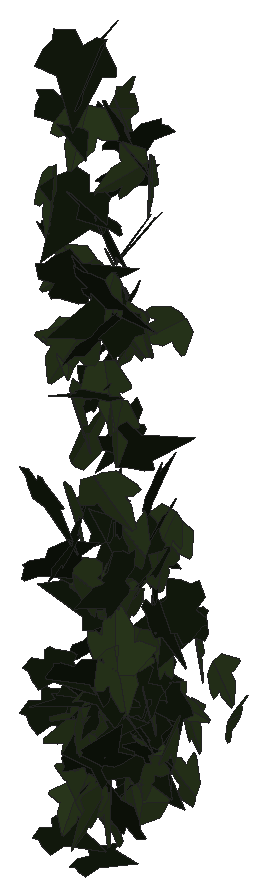
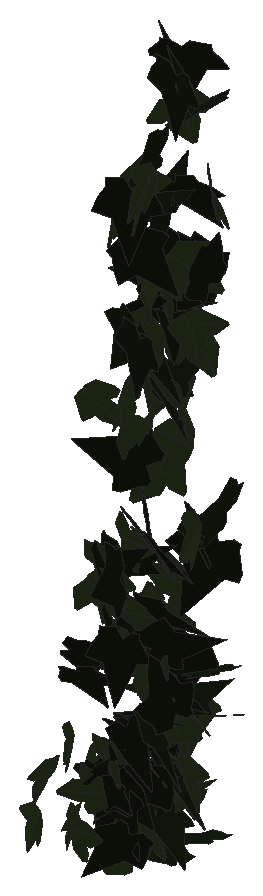
# SketchUp Ruby script. Lengths in inches.
U = 1.inch
M = Sketchup.active_model
def pt(a) = Geom::Point3d.new(a.map { |v| v * U })
def face(e, loops, mat)
  f = e.add_face(loops[0].map { |a| pt(a) })
  loops[1..].each { |l| e.add_face(l.map { |a| pt(a) }).erase! }
  f.material = f.back_material = mat if mat
  f
end
# faces: each face lists its corners as indices into pts; further lists are holes
def faces(e, pts, list, mat = nil) = list.each { |f| face(e, (f[0].is_a?(Array) ? f : [f]).map { |l| l.map { |i| pts[i] } }, mat) }
# xy, xz, yz: faces in a plane at the given z, y or x. An outline is a flat list of corners, or four numbers for a rectangle; further outlines are holes
def ring(l) = l.size == 4 ? [[l[0], l[1]], [l[2], l[1]], [l[2], l[3]], [l[0], l[3]]] : l.each_slice(2).to_a
def flat(e, list, mat, &to3) = list.each { |f| face(e, (f[0].is_a?(Array) ? f : [f]).map { |l| ring(l).map { |u, v| to3.(u, v) } }, mat) }
def xy(e, z, list, mat = nil) = flat(e, list, mat) { |x, y| [x, y, z] }
def xz(e, y, list, mat = nil) = flat(e, list, mat) { |x, z| [x, y, z] }
def yz(e, x, list, mat = nil) = flat(e, list, mat) { |y, z| [x, y, z] }
def lines(e, pts, list) = list.each { |a, b| e.add_line(pt(pts[a]), pt(pts[b])) }
# prism: a flat outline (further loops are holes) pulled along v
def prism(e, loops, v, mat = nil)
  f = face(e, loops, mat); d = Geom::Vector3d.new(v.map { |x| x * U })
  f.pushpull(f.normal.samedirection?(d) ? d.length : -d.length)
end
def box(e, o, s, mat = nil) = prism(e, [[o, [o[0] + s[0], o[1], o[2]], [o[0] + s[0], o[1] + s[1], o[2]], [o[0], o[1] + s[1], o[2]]]], [0, 0, s[2]], mat)
def at(x, y, z, deg = 0) = Geom::Transformation.translation(pt([x, y, z])) * Geom::Transformation.rotation(ORIGIN, Z_AXIS, deg.degrees)
def axes(o, x, y, z) = Geom::Transformation.new([*x, 0, *y, 0, *z, 0, *pt(o).to_a, 1])
def part(name) = M.definitions.add(name)
# library, detail: a bought-in or finely detailed component or shape, given as its bounding box
def library(name, o, s) = part(name).tap { |d| box(d.entities, o, s) }
def detail(e, o, s) = box(e.add_group.entities, o, s)
def put(e, d, t, mat = nil) = e.add_instance(d, t).tap { |i| i.material = mat if mat }
def group(e, t, mat = nil) = e.add_group.tap { |g| g.transformation = t; g.material = mat if mat }.entities
root = M.entities
M.materials.add("efeu1").color = [18, 25, 13]
M.materials.add("efeu2").color = [43, 57, 29]
c1 = part("ivyleaf_9")
p = [[1.54,2.16,1.25],[1.36,2.04,1.19],[-0.21,0.99,0.68],[-0.71,1.11,0.82],[-0.85,0.86,0.67],[-0.8,0.17,0.21],
  [-0.9,-0.01,0.1],[-0.67,-0.16,-0.02],[-0.08,-0.08,-0.05],[-0.03,-0.6,-0.4],[0.65,-0.88,-0.66],[0.83,-0.6,-0.49],
  [1.29,-0.42,-0.43],[1.8125,-0.07,-0.26],[1.21,0.44,0.15]]
faces(c1.entities,p,[[0,1,2,3,4,5,6,7,8,9,10,11,12,13,14]],"efeu1")
c2 = part("ivyleaf_10")
p = [[0,0.5,-0.03],[-0.0625,2.02,-0.43],[-0.19,2.01,-0.46],[-0.54,1.05,-0.29],[-0.52,0.625,-0.18],[-0.83,0.76,-0.28],
  [-1.16,0.64,-0.33],[-1.15,0.33,-0.24],[-0.77,-0.39,0.02],[-0.3,-0.51,0.16],[0.04,-0.48,0.23],[-0.02,2.01,-0.4375],
  [-0.06,2.01,-0.43],[0.04,-0.49,0.23],[0.67,-0.49,0.14],[1.38,0.36,-0.2],[1.375,0.51,-0.24],[0.81,0.65,-0.19],
  [0.62,0.59,-0.15],[0.6,1.09,-0.28],[0.5,1.23,-0.31]]
faces(c2.entities,p,[[0,1,2,3,4,5,6,7,8,9,10],[11,12,0,13,14,15,16,17,18,19,20]],"efeu2")
put(root,c1,axes([591.08,128.32,222.35],[0.71434,-0.84859,0.27157],[0.2006,-0.18596,-1.10875],[0.86811,0.74125,0.03274]))
put(root,c1,axes([592.37,131.6,213.37],[-0.64879,0.80027,0.11498],[-0.05608,0.10253,-1.03001],[-0.80654,-0.65087,-0.02088]))
put(root,c1,axes([592.22,132.46,231.86],[-0.1377,0.87962,0.41752],[-0.02989,0.41766,-0.88977],[-0.97322,-0.13729,-0.03175]))
put(root,c1,axes([592.39,132.84,223.6],[-0.90047,0.24398,-0.18064],[0.17365,-0.04982,-0.93294],[-0.249,-0.91706,0.00263]))
put(root,c1,axes([592.79,130.74,216.47],[-0.38209,-0.03827,0.95633],[-0.9535,-0.07396,-0.38392],[0.08289,-1.02718,-0.00799]))
put(root,c2,axes([591.83,129.36,221.66],[-0.68075,0.69399,-0.45796],[0.31524,-0.33227,-0.9721],[-0.7694,-0.75016,0.00691]))
put(root,c1,axes([591.75,130.83,213.9],[0.53956,0.76186,0.30871],[-0.17431,-0.25483,0.93356],[0.80333,-0.567,-0.00478]))
put(root,c1,axes([591.49,128.09,212.58],[0.45938,-0.62897,-0.3329],[0.42232,0.55986,-0.47503],[0.57277,0.09165,0.61724]))
put(root,c2,axes([592.44,131.87,238.72],[-0.59711,0.70119,0.36728],[-0.21514,0.29898,-0.92055],[-0.76176,-0.63407,-0.02791]))
put(root,c1,axes([592.61,132.75,213.55],[-0.28986,0.78694,-0.427],[0.15143,-0.39926,-0.83862],[-0.88242,-0.32701,-0.00365]))
put(root,c2,axes([592.51,131.53,238.79],[-0.00324,0.42152,0.9162],[-0.394,0.84286,-0.38918],[-0.92837,-0.35918,0.16197]))
put(root,c1,axes([591.68,128.05,214.57],[0.46653,-0.69067,-0.20201],[0.43037,0.46074,-0.58136],[0.57673,0.21488,0.59724]))
put(root,c2,axes([591.93,127.91,236.875],[0.78499,-0.50136,0.6475],[0.53824,-0.36012,-0.93137],[0.61719,0.95173,-0.01132]))
put(root,c1,axes([592.59,132.39,232.125],[0.19052,0.67199,0.69095],[-0.02852,0.70794,-0.68065],[-0.96341,0.11193,0.15679]))
put(root,c1,axes([591.66,128.67,233.23],[0.21748,-0.4109,0.99451],[0.61968,-0.78166,-0.45847],[0.87971,0.6522,0.0771]))
put(root,c1,axes([592.4,127.22,219.93],[0.56944,1.01131,0.19538],[0.09984,0.16801,-1.1606],[-1.02516,0.57811,-0.0045]))
put(root,c1,axes([592.94,131.88,235.92],[-0.26019,0.66153,-0.69309],[-0.06823,-0.72916,-0.67034],[-0.95569,-0.12804,0.23656]))
put(root,c1,axes([592.61,133.14,217.86],[0.64515,0.47543,-0.46119],[-0.36967,-0.27578,-0.8014],[-0.54962,0.74355,-0.00234]))
put(root,c1,axes([591.85,128.34,206.78],[0.52205,-0.62356,-0.13993],[0.45754,0.49084,-0.48028],[0.44616,0.22626,0.65627]))
put(root,c1,axes([592.95,129.2,242.53],[-0.12779,0.96242,0.39875],[-0.10849,0.38726,-0.96946],[-1.03609,-0.15925,0.05233]))
put(root,c2,axes([592.59,132.96,227.91],[-0.16116,0.4278,-0.84597],[-0.16409,-0.85775,-0.40249],[-0.93368,0.0769,0.21676]))
put(root,c1,axes([593.32,130.15,220.66],[-0.45039,0.48984,0.72061],[-0.55237,0.46684,-0.66258],[-0.67387,-0.71006,0.06149]))
put(root,c1,axes([593.39,130.39,217.93],[-0.70295,0.2422,0.61954],[-0.61174,0.11866,-0.74049],[-0.26128,-0.92946,0.06691]))
put(root,c1,axes([593.06,128.63,213.02],[-0.82697,-0.14019,-0.01774],[0.13742,-0.7733,-0.29491],[0.03293,-0.2936,0.78522]))
put(root,c2,axes([593.37,128.4,233.35],[-0.37147,-0.48566,0.8732],[-0.55618,-0.67341,-0.61115],[0.83006,-0.66856,-0.01873]))
put(root,c2,axes([593.25,130.65,214.36],[-0.86499,0.13063,-0.387],[-0.37881,0.0824,0.8745],[0.15276,0.94403,-0.02278]))
put(root,c2,axes([592.65,128.34,230.04],[-0.27489,-0.83563,0.3812],[0.43865,-0.46903,-0.71186],[0.80695,-0.02969,0.51682]))
put(root,c1,axes([593.45,129.23,210.21],[-0.79682,0.75112,-0.0469],[0.01627,-0.0511,-1.09472],[-0.7524,-0.79656,0.026]))
put(root,c1,axes([593.58,129.09,227.27],[-0.33431,0.68735,0.69702],[-0.39401,0.57977,-0.76071],[-0.89613,-0.51134,0.07444]))
put(root,c1,axes([592.52,128.61,212.69],[0.83419,0.01828,-0.07269],[0.00581,0.79408,0.26627],[0.07473,-0.26571,0.79076]))
put(root,c2,axes([593.38,127.78,230],[-0.74645,-0.63996,0.55279],[-0.37494,-0.41045,-0.98146],[0.75799,-0.83325,0.0589]))
put(root,c1,axes([593.6,129.42,208.13],[-0.23645,1.04066,0.13985],[-0.38471,0.04753,-1.00408],[-0.977,-0.27057,0.36153]))
put(root,c2,axes([593.05,133.72,213.07],[0.8384,-0.30904,-0.2059],[-0.18613,0.09021,-0.89333],[0.32133,0.85859,0.01975]))
put(root,c2,axes([592.85,128.4,208.54],[-0.4072,-0.49071,0.53152],[0.32831,-0.66887,-0.366],[0.64461,0.03068,0.52217]))
put(root,c1,axes([593.22,127.12,220.12],[-0.58961,0.71077,-0.37211],[-0.30652,0.22718,0.91964],[0.74142,0.65916,0.08428]))
put(root,c2,axes([593.76,129.74,217.38],[0.06324,0.05747,1.00865],[-0.95957,-0.31278,0.07798],[0.31609,-0.96101,0.03493]))
put(root,c2,axes([593.49,128.34,209.5],[-0.97588,-0.08078,0.50102],[-0.47157,-0.25696,-0.95994],[0.18755,-1.06646,0.19335]))
put(root,c1,axes([593.22,132.5625,220.3],[0.05258,0.34053,1.03455],[0.17075,1.02037,-0.34454],[-1.07569,0.17861,-0.00412]))
put(root,c1,axes([593.25,134.03,211.85],[-0.40091,-0.50236,0.61577],[-0.26079,-0.56833,-0.63345],[0.75068,-0.46573,0.1088]))
put(root,c2,axes([593.11,128.88,211.76],[-0.81701,-0.78336,0.02363],[0.03671,-0.00416,1.13153],[-0.78286,0.81734,0.0284]))
put(root,c1,axes([593.35,131.5625,237.98],[0.30137,0.92296,-0.24577],[-0.08305,-0.23142,-0.97089],[-0.9515,0.31253,0.0069]))
put(root,c1,axes([592.61,128.06,240.625],[0.10976,-1.00353,0.13731],[0.45467,-0.0746,-0.90867],[0.9051,0.15917,0.43981]))
put(root,c2,axes([593.34,128.25,224.75],[0.28069,-0.75968,0.88908],[-0.26888,0.84791,0.80939],[-1.1381,-0.38768,0.02805]))
put(root,c1,axes([592.92,132.39,208.3],[-0.09057,-0.26221,-0.88706],[0.28253,0.84086,-0.2774],[0.88079,-0.29669,-0.00224]))
put(root,c2,axes([593.3125,127.91,227.16],[-0.67443,0.96065,0.08902],[-0.03765,0.08233,-1.17364],[-0.96403,-0.67528,-0.01644]))
put(root,c2,axes([593.99,129.59,207.1875],[-0.24981,0.08231,0.88203],[-0.84358,0.25766,-0.26296],[-0.27043,-0.87977,0.00551]))
put(root,c1,axes([592.58,127.67,232.52],[0.42198,0.05857,1.04073],[1.02374,0.18805,-0.42568],[-0.1962,1.10717,0.01724]))
put(root,c2,axes([593.61,127.875,212.25],[-0.52802,-0.96958,0.06158],[-0.03392,-0.05165,-1.10402],[0.97094,-0.52908,-0.00508]))
put(root,c1,axes([593.7,128.09,236.76],[-1.02962,-0.46391,-0.08687],[0.07985,0.03424,-1.12931],[0.46517,-1.03271,0.00158]))
put(root,c1,axes([593.49,127.67,215.03],[0.64517,0.78827,-0.27102],[-0.18198,-0.20124,-1.01855],[-0.81345,0.67022,0.01291]))
put(root,c1,axes([594.21,128.06,213.14],[-0.65183,0.66921,0.43797],[-0.35893,0.26014,-0.93169],[-0.71473,-0.74097,0.06846]))
put(root,c2,axes([593.39,131.72,228.94],[0.20807,-0.81917,-0.35874],[0.24768,0.4067,-0.78503],[0.85929,0.08112,0.31314]))
put(root,c1,axes([593.98,131.48,212.79],[-1.02357,-0.15606,0.08121],[-0.0597,-0.14286,-1.02698],[0.16549,-1.0168,0.13182]))
put(root,c1,axes([593.39,128.19,243.32],[-0.76281,-0.68855,-0.51611],[0.38968,0.33852,-1.02757],[0.76721,-0.85653,0.00877]))
put(root,c1,axes([594,131.75,209.4],[0.3317,0.30094,-0.80444],[-0.70365,-0.39929,-0.43951],[-0.49252,0.77313,0.08614]))
put(root,c1,axes([593.87,132.02,210.51],[-0.10063,0.56751,-0.79428],[0.04409,-0.79503,-0.57363],[-0.9752,-0.09451,0.05603]))
put(root,c1,axes([593.26,127.97,241.26],[-0.16158,0.87463,0.66358],[0.12888,-0.65098,0.88941],[1.09028,0.20657,-0.00679]))
put(root,c1,axes([593.08,130.26,239.3],[0.88584,-0.62923,-0.08232],[-0.06237,0.05434,-1.08654],[0.63152,0.88799,0.00816]))
put(root,c2,axes([593.81,130.65,210.42],[-0.8097,-0.12288,0.06986],[-0.06923,-0.00947,-0.81897],[0.12324,-0.81266,-0.00102]))
put(root,c1,axes([594.05,131.25,212.26],[-0.78015,0.25614,-0.10132],[0.09013,-0.05019,-0.82089],[-0.26029,-0.7851,0.01942]))
put(root,c1,axes([594.07,130.04,230.62],[-0.85623,0.78935,-0.53568],[0.39855,-0.35798,-1.16454],[-0.86671,-0.94442,-0.0063]))
put(root,c1,axes([593.15,131.22,210.8],[-0.3106,-0.51139,-1.10038],[0.54288,0.95727,-0.59812],[1.08519,-0.62525,-0.01573]))
put(root,c2,axes([593.91,132.29,207.02],[0.06949,0.22117,0.93813],[-0.17195,-0.92264,0.23025],[0.94839,-0.18349,-0.02699]))
put(root,c2,axes([593.79,131.46,208.16],[-0.10342,-0.78515,-0.14467],[0.02905,0.14208,-0.79187],[0.79784,-0.10695,0.01008]))
put(root,c2,axes([593.8,127.88,212.63],[-0.20062,1.04503,0.32623],[-0.21147,0.28842,-1.05397],[-1.07415,-0.25197,0.14656]))
put(root,c2,axes([594.25,133.07,228.82],[0.55575,0.13983,-0.73669],[-0.74536,0.00289,-0.56174],[-0.08188,0.9228,0.11339]))
put(root,c1,axes([593.48,133.37,211.27],[-0.67095,-0.28649,-0.81053],[0.74704,0.31448,-0.72955],[0.4254,-1.00411,0.00277]))
put(root,c2,axes([593.79,127.84,240.41],[0.72908,0.76062,-0.27727],[-0.20791,-0.18471,-1.05339],[-0.78243,0.75784,0.02155]))
put(root,c2,axes([593.59,130.22,217.42],[-0.05046,-0.50908,0.85746],[0.15352,0.84436,0.51034],[-0.98531,0.15763,0.0356]))
put(root,c1,axes([593.63,128.72,210.98],[0.57862,-0.71476,-0.53919],[0.33528,-0.42229,0.9196],[-0.83018,-0.66872,-0.00441]))
put(root,c2,axes([593.07,128.74,218.5],[-0.15302,0.10894,-1.11588],[0.99716,-0.50166,-0.18572],[-0.51258,-1.00844,-0.02816]))
put(root,c1,axes([593.21,128.99,205.69],[0.46303,-0.6472,0.03496],[0.6141,0.42432,-0.27806],[0.2073,0.18859,0.74561]))
put(root,c1,axes([593.28,128.78,211.77],[0.72179,-0.26233,-0.32377],[0.26977,0.78771,-0.03683],[0.3176,-0.0729,0.7671]))
put(root,c1,axes([594.32,130.72,217.73],[-0.46519,0.72524,0.02949],[-0.00256,0.03338,-0.86146],[-0.72583,-0.46492,-0.01586]))
put(root,c2,axes([593.92,134.48,210.05],[-0.29022,0.8146,0.11247],[-0.04921,0.10185,-0.86467],[-0.82085,-0.29412,0.01207]))
put(root,c2,axes([593.79,130.29,212.53],[0.58167,-0.52113,0.2878],[0.26694,-0.13133,-0.77732],[0.53211,0.63554,0.07536]))
put(root,c2,axes([594.18,130.97,209.49],[-0.81846,-0.50642,0.01917],[-0.01622,-0.01021,-0.96246],[0.50652,-0.81862,0.00015]))
put(root,c1,axes([594.34,128.53,227.54],[-0.90132,-0.15424,-0.00056],[0.15076,-0.88028,-0.19636],[0.03258,-0.19364,0.89309]))
put(root,c2,axes([593.95,130.68,208.55],[-0.18284,0.78758,-0.03931],[0.01876,-0.036,-0.80846],[-0.78833,-0.18352,-0.01012]))
put(root,c2,axes([593.94,131.46,209.99],[0.70481,0.41027,0.01264],[0.01081,0.00655,-0.81552],[-0.41032,0.7049,0.00022]))
put(root,c2,axes([593.99,128.44,208.72],[0.24585,-0.65126,0.83246],[0.24515,-0.79624,-0.69532],[1.02812,0.34559,-0.03327]))
put(root,c2,axes([593.43,133.83,210.82],[0.17663,0.03919,0.87551],[0.81211,0.32841,-0.17854],[-0.32944,0.83058,0.02929]))
put(root,c2,axes([593.51,130.12,232.2],[-0.20877,-0.17529,0.98399],[0.91039,-0.44822,0.11331],[0.4125,0.90051,0.24794]))
put(root,c1,axes([594.02,130.06,210.34],[0.60093,0.55904,0.02959],[0.01945,0.02253,-0.82075],[-0.55949,0.60123,0.00325]))
put(root,c2,axes([594.25,130.1875,217.32],[0.02677,-1.03174,0.3227],[0.01894,-0.3223,-1.03204],[1.08086,0.0312,0.01009]))
put(root,c1,axes([594.82,130.44,219.61],[-0.66599,-0.63814,-0.34944],[-0.25339,-0.24063,0.92237],[-0.682,0.71257,-0.00146]))
put(root,c2,axes([594.14,131.42,212.32],[-0.4252,0.71134,-0.02644],[0.01711,-0.02058,-0.82872],[-0.71163,-0.42552,-0.00412]))
put(root,c2,axes([594.02,134.81,213.49],[-0.49941,0.58873,-0.41896],[0.19579,-0.37999,-0.76734],[-0.69556,-0.52967,0.08482]))
put(root,c1,axes([594.5,131.5,217.23],[0.17429,-0.09987,1.01396],[-0.04995,1.02662,0.1097],[-1.01764,-0.06749,0.16827]))
put(root,c2,axes([593.79,129.08,228],[1.01159,-0.02279,0.45663],[0.45719,0.05924,-1.00986],[-0.00363,1.1083,0.06337]))
put(root,c2,axes([593.92,129.8125,230.62],[-0.86192,0.07026,-0.57313],[0.56746,-0.08745,-0.8641],[-0.10683,-1.03138,0.03423]))
put(root,c1,axes([593.93,129.79,221.41],[-0.09314,0.39556,0.91782],[0.18806,-0.8984,0.40627],[0.98158,0.20966,0.00925]))
put(root,c1,axes([594.22,128.25,235.66],[0.84274,-0.25468,-0.66578],[-0.62574,0.22948,-0.87984],[0.34143,1.0492,0.03083]))
put(root,c2,axes([594.41,130.3125,237.27],[0.03076,-0.13636,1.04254],[0.0433,-1.04194,-0.13755],[1.05053,0.04694,-0.02485]))
put(root,c2,axes([594.6,132.5625,219.62],[0.47725,0.49761,-0.62637],[-0.51586,-0.36602,-0.68383],[-0.61142,0.69723,0.08804]))
put(root,c2,axes([594.19,129.55,226.17],[-0.11012,0.92953,-0.41055],[0.05872,-0.40644,-0.93598],[-1.01446,-0.12443,-0.00961]))
put(root,c1,axes([594.77,128.94,231.4],[-0.0428,-0.39228,-1.00743],[-0.1491,-0.99644,0.39433],[-1.07077,0.15443,-0.01465]))
put(root,c2,axes([594.32,128.65,232.54],[1.04563,-0.38425,-0.06456],[-0.05744,0.03085,-1.11396],[0.38538,1.04716,0.00913]))
put(root,c1,axes([594.39,130.14,210.31],[-0.30694,-0.49467,0.57892],[-0.19117,-0.55413,-0.57485],[0.73709,-0.34971,0.09198]))
put(root,c1,axes([593.86,127.87,210.625],[0.79671,0.72863,0.15584],[-0.11662,-0.1034,1.07965],[0.73593,-0.80519,0.00238]))
put(root,c1,axes([594.25,128.46,235.84],[-0.59761,-0.42842,0.61434],[0.31785,-0.85673,-0.28826],[0.67819,0.024,0.67645]))
put(root,c1,axes([594.8,127.04,231.07],[-0.05859,1.13142,0.11503],[-0.02484,0.11388,-1.13278],[-1.13698,-0.06079,0.01882]))
put(root,c2,axes([595.12,129.75,220.25],[0.30895,0.01976,0.98603],[-0.9799,0.12298,0.30456],[-0.11151,-1.02595,0.0555]))
put(root,c2,axes([594.33,131.5,236.71],[-0.43056,0.71184,-0.53932],[0.08676,-0.56255,-0.81177],[-0.88885,-0.39972,0.18201]))
put(root,c1,axes([594.89,131.58,219.39],[-0.79344,0.44652,-0.24356],[0.20563,-0.13117,-0.91036],[-0.4652,-0.81955,0.01301]))
put(root,c2,axes([594.78,130.04,215.95],[-0.62337,-0.51256,0.27435],[-0.15011,-0.2467,-0.80199],[0.56165,-0.63482,0.09016]))
put(root,c1,axes([594.97,128.9,207.87],[0.49766,-0.53713,0.87346],[-0.60845,0.62681,0.73212],[-0.82537,-0.78594,-0.01305]))
put(root,c1,axes([594.14,129.13,213.4],[-0.2081,-0.79448,0.17405],[0.58376,-0.27099,-0.53905],[0.56631,-0.0126,0.61962]))
put(root,c2,axes([595.25,132.86,207.9],[0.29539,-0.03577,0.93929],[-0.93397,0.09987,0.29752],[-0.10601,-0.97956,-0.00396]))
put(root,c2,axes([594.6,128.88,215.37],[1.17088,0.29132,0.10886],[-0.10905,-0.01252,1.20649],[0.29124,-1.17586,0.01412]))
put(root,c1,axes([594.82,133.25,215.71],[-0.79023,-0.4265,-0.15279],[0.13533,0.07096,-0.89798],[0.43236,-0.80173,0.00181]))
put(root,c1,axes([594.93,131.48,220.78],[-0.50725,0.55532,-0.44147],[0.30304,-0.32108,-0.7521],[-0.64144,-0.59085,-0.00621]))
put(root,c2,axes([594.44,128.22,223.56],[-0.96173,-0.2443,-0.53757],[0.53453,0.07633,-0.99098],[0.25088,-1.09913,0.05066]))
put(root,c1,axes([594.17,130.29,211.875],[0.2868,-0.56189,0.53665],[0.3667,-0.40644,-0.62154],[0.68502,0.45283,0.10804]))
put(root,c1,axes([595.48,128.19,219.52],[-0.89406,0.55615,0.13958],[-0.13009,0.05508,-1.0527],[-0.55845,-0.90321,0.02175]))
put(root,c1,axes([595.48,132.69,216.23],[-0.81419,-0.05907,0.46775],[-0.46626,-0.03752,-0.81632],[0.06991,-0.93824,0.00319]))
put(root,c1,axes([594.47,131.5,216.4],[0.65578,-0.62001,-0.26629],[-0.19629,0.18,-0.90247],[0.6456,0.68452,-0.00389]))
put(root,c2,axes([594.93,131.15,219.04],[-0.37084,-0.77373,-0.1068],[0.07264,0.08355,-0.85751],[0.77768,-0.37676,0.02917]))
put(root,c1,axes([594.11,129.85,224.26],[0.36466,-0.08386,0.99699],[0.99604,0.13063,-0.35333],[-0.09448,1.05352,0.12317]))
put(root,c2,axes([594.44,128.49,209.3],[0.63529,-0.51014,0.71497],[0.62767,-0.35354,-0.80997],[0.61437,0.8887,0.08819]))
put(root,c2,axes([595.21,135.56,209.71],[0.13249,0.33771,0.74564],[-0.50102,0.63078,-0.19666],[-0.6473,-0.41911,0.30484]))
put(root,c2,axes([594.86,135.125,212.125],[-0.08298,0.82646,0.24025],[-0.00109,0.24126,-0.83032],[-0.86067,-0.07999,-0.02211]))
put(root,c1,axes([594.01,127.98,232.55],[0.85623,-0.37304,0.70548],[0.64084,-0.29525,-0.93389],[0.4756,1.06942,-0.01174]))
put(root,c2,axes([594.79,128.68,215.38],[0.3452,1.0868,0.09367],[0.02629,0.08993,-1.1403],[-1.09051,0.34619,0.00216]))
put(root,c2,axes([595.07,131.72,220.62],[0.80774,-0.23669,-0.22798],[-0.20199,0.11962,-0.83984],[0.25922,0.83073,0.05597]))
put(root,c2,axes([594.93,132.26,210.52],[-0.14623,0.19943,-0.87488],[0.07886,-0.88014,-0.21381],[-0.89385,-0.11027,0.12426]))
